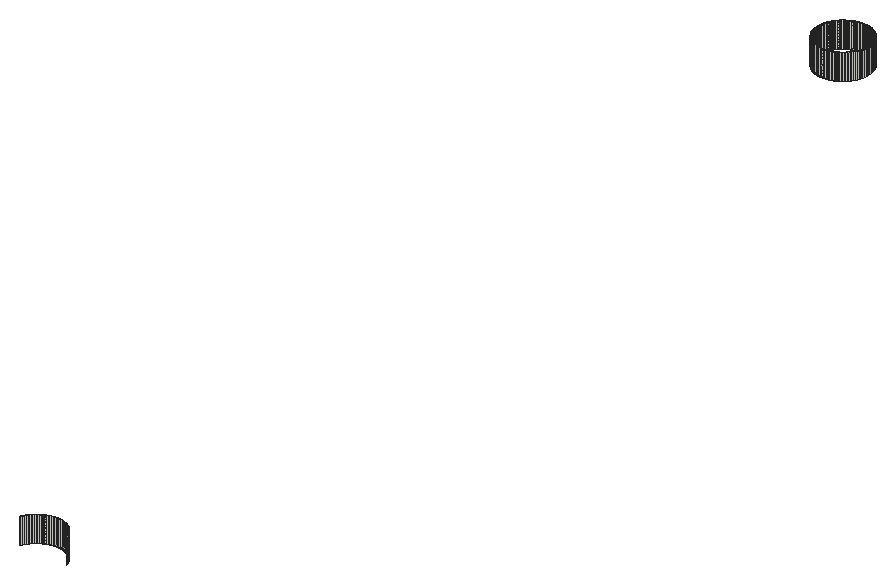
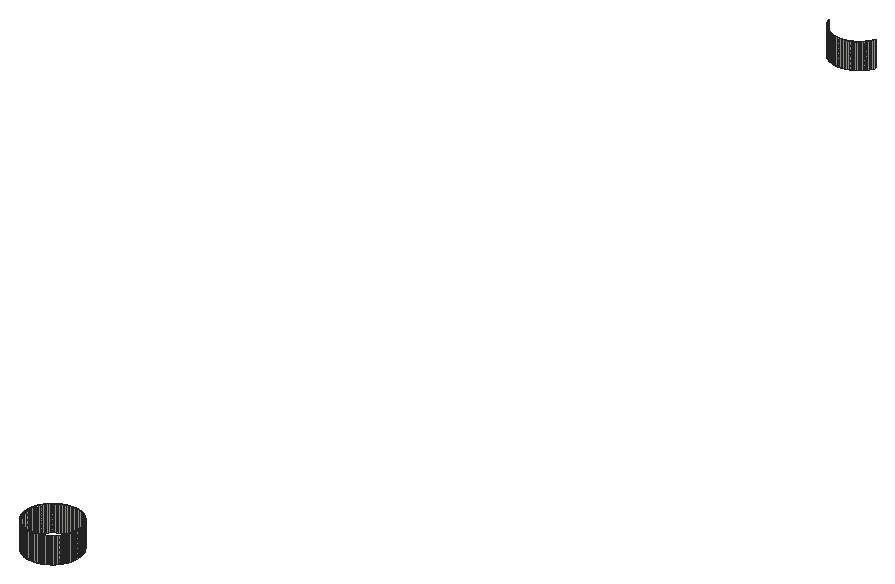
# SketchUp Ruby script. Lengths in inches.
U = 1.inch
M = Sketchup.active_model
def pt(a) = Geom::Point3d.new(a.map { |v| v * U })
def face(e, loops, mat)
  f = e.add_face(loops[0].map { |a| pt(a) })
  loops[1..].each { |l| e.add_face(l.map { |a| pt(a) }).erase! }
  f.material = f.back_material = mat if mat
  f
end
# faces: each face lists its corners as indices into pts; further lists are holes
def faces(e, pts, list, mat = nil) = list.each { |f| face(e, (f[0].is_a?(Array) ? f : [f]).map { |l| l.map { |i| pts[i] } }, mat) }
# xy, xz, yz: faces in a plane at the given z, y or x. An outline is a flat list of corners, or four numbers for a rectangle; further outlines are holes
def ring(l) = l.size == 4 ? [[l[0], l[1]], [l[2], l[1]], [l[2], l[3]], [l[0], l[3]]] : l.each_slice(2).to_a
def flat(e, list, mat, &to3) = list.each { |f| face(e, (f[0].is_a?(Array) ? f : [f]).map { |l| ring(l).map { |u, v| to3.(u, v) } }, mat) }
def xy(e, z, list, mat = nil) = flat(e, list, mat) { |x, y| [x, y, z] }
def xz(e, y, list, mat = nil) = flat(e, list, mat) { |x, z| [x, y, z] }
def yz(e, x, list, mat = nil) = flat(e, list, mat) { |y, z| [x, y, z] }
def lines(e, pts, list) = list.each { |a, b| e.add_line(pt(pts[a]), pt(pts[b])) }
# prism: a flat outline (further loops are holes) pulled along v
def prism(e, loops, v, mat = nil)
  f = face(e, loops, mat); d = Geom::Vector3d.new(v.map { |x| x * U })
  f.pushpull(f.normal.samedirection?(d) ? d.length : -d.length)
end
def box(e, o, s, mat = nil) = prism(e, [[o, [o[0] + s[0], o[1], o[2]], [o[0] + s[0], o[1] + s[1], o[2]], [o[0], o[1] + s[1], o[2]]]], [0, 0, s[2]], mat)
def at(x, y, z, deg = 0) = Geom::Transformation.translation(pt([x, y, z])) * Geom::Transformation.rotation(ORIGIN, Z_AXIS, deg.degrees)
def axes(o, x, y, z) = Geom::Transformation.new([*x, 0, *y, 0, *z, 0, *pt(o).to_a, 1])
def part(name) = M.definitions.add(name)
# library, detail: a bought-in or finely detailed component or shape, given as its bounding box
def library(name, o, s) = part(name).tap { |d| box(d.entities, o, s) }
def detail(e, o, s) = box(e.add_group.entities, o, s)
def put(e, d, t, mat = nil) = e.add_instance(d, t).tap { |i| i.material = mat if mat }
def group(e, t, mat = nil) = e.add_group.tap { |g| g.transformation = t; g.material = mat if mat }.entities
root = M.entities
xz(root,416.82,[[28.6875,258,28.76,261],[29.24,258,29.3125,261]])
xz(root,416.83,[[28.84,258,28.92,261],[28.92,258,29,261],[29,258,29.08,261],[29.08,258,29.16,261]])
xz(root,529,[[28.84,258,28.92,261],[28.92,258,29,261],[29,258,29.08,261],[29.08,258,29.16,261]])
xz(root,535,[[28.84,258,28.92,261],[28.92,258,29,261],[29,258,29.08,261],[29.08,258,29.16,261]])
yz(root,26,[[531.84,258,531.92,261],[531.92,258,532,261],[532,258,532.08,261],[532.08,258,532.16,261]])
yz(root,32,[[531.84,258,531.92,261],[531.92,258,532,261],[532,258,532.08,261],[532.08,258,532.16,261]])
p = [[31.8,414.91,258],[31.83,414.83,258],[31.83,414.83,261],[31.8,414.91,261],[26.2,414.91,258],[26.23,414.98,258],
  [26.23,414.98,261],[26.2,414.91,261],[31.77,414.98,258],[31.77,414.98,261],[26.26,415.05,258],[26.26,415.05,261],
  [31.74,415.05,258],[31.74,415.05,261],[26.29,415.125,258],[26.29,415.125,261],[26.33,415.2,258],[26.33,415.2,261],
  [31.71,415.125,258],[31.71,415.125,261],[31.67,415.2,258],[31.67,415.2,261],[26.36,415.26,258],[26.36,415.26,261],
  [31.64,415.26,258],[31.64,415.26,261],[26.4,415.33,258],[26.4,415.33,261],[26.44,415.4,258],[26.44,415.4,261],
  [31.6,415.33,258],[31.6,415.33,261],[31.56,415.4,258],[31.56,415.4,261],[26.48,415.47,258],[26.48,415.47,261],
  [31.52,415.47,258],[31.52,415.47,261],[26.53,415.53,258],[26.53,415.53,261],[26.57,415.6,258],[26.57,415.6,261],
  [31.43,415.6,258],[31.47,415.53,258],[31.47,415.53,261],[31.43,415.6,261],[26.62,415.66,258],[26.62,415.66,261],
  [31.38,415.66,258],[31.38,415.66,261],[26.67,415.72,258],[26.67,415.72,261],[26.72,415.78,258],[26.72,415.78,261],
  [31.33,415.72,258],[31.33,415.72,261],[31.28,415.78,258],[31.28,415.78,261],[26.77,415.84,258],[26.77,415.84,261],
  [26.82,415.9,258],[26.82,415.9,261],[31.23,415.84,258],[31.23,415.84,261],[31.18,415.9,258],[31.18,415.9,261],
  [26.88,415.95,258],[26.88,415.95,261],[31.12,415.95,258],[31.12,415.95,261],[26.93,416.01,258],[26.93,416.01,261],
  [26.99,416.0625,258],[26.99,416.0625,261],[31.01,416.0625,258],[31.07,416.01,258],[31.07,416.01,261],[31.01,416.0625,261],
  [27.05,416.11,258],[27.05,416.11,261],[27.11,416.16,258],[27.11,416.16,261],[30.95,416.11,258],[30.95,416.11,261],
  [30.89,416.16,258],[30.89,416.16,261],[27.17,416.21,258],[27.17,416.21,261],[27.24,416.26,258],[27.24,416.26,261],
  [30.83,416.21,258],[30.83,416.21,261],[30.76,416.26,258],[30.76,416.26,261],[27.3,416.31,258],[27.3,416.31,261],
  [27.37,416.35,258],[27.37,416.35,261],[27.43,416.39,258],[27.43,416.39,261],[30.63,416.35,258],[30.7,416.31,258],
  [30.7,416.31,261],[30.63,416.35,261],[30.57,416.39,258],[30.57,416.39,261],[27.5,416.43,258],[27.5,416.43,261],
  [27.57,416.47,258],[27.57,416.47,261],[30.43,416.47,258],[30.5,416.43,258],[30.5,416.43,261],[30.43,416.47,261],
  [27.64,416.51,258],[27.64,416.51,261],[27.71,416.54,258],[27.71,416.54,261],[27.78,416.57,258],[27.78,416.57,261],
  [30.22,416.57,258],[30.29,416.54,258],[30.29,416.54,261],[30.22,416.57,261],[30.36,416.51,258],[30.36,416.51,261],
  [27.85,416.6,258],[27.85,416.6,261],[27.92,416.63,258],[27.92,416.63,261],[28,416.66,258],[28,416.66,261],
  [30,416.66,258],[30.08,416.63,258],[30.08,416.63,261],[30,416.66,261],[30.15,416.6,258],[30.15,416.6,261],
  [28.07,416.6875,258],[28.07,416.6875,261],[28.15,416.71,258],[28.15,416.71,261],[28.22,416.73,258],[28.22,416.73,261],
  [28.3,416.75,258],[28.3,416.75,261],[29.7,416.75,258],[29.78,416.73,258],[29.78,416.73,261],[29.7,416.75,261],
  [29.85,416.71,258],[29.85,416.71,261],[29.93,416.6875,258],[29.93,416.6875,261],[28.375,416.77,258],[28.375,416.77,261],
  [28.45,416.78,258],[28.45,416.78,261],[28.53,416.8,258],[28.53,416.8,261],[28.61,416.81,258],[28.61,416.81,261],
  [28.6875,416.82,258],[28.6875,416.82,261],[28.76,416.82,258],[28.84,416.83,258],[28.84,416.83,261],[28.76,416.82,261],
  [29.16,416.83,258],[29.24,416.82,258],[29.24,416.82,261],[29.16,416.83,261],[29.3125,416.82,258],[29.39,416.81,258],
  [29.39,416.81,261],[29.3125,416.82,261],[29.47,416.8,258],[29.47,416.8,261],[29.55,416.78,258],[29.625,416.77,258],
  [29.625,416.77,261],[29.55,416.78,261],[28.61,529.03,258],[28.53,529.04,258],[28.53,529.04,261],[28.61,529.03,261],
  [28.45,529.05,258],[28.45,529.05,261],[28.6875,529.02,258],[28.6875,529.02,261],[28.76,529.01,258],[28.76,529.01,261],
  [28.84,529,258],[28.84,529,261],[29.24,529.01,258],[29.16,529,258],[29.16,529,261],[29.24,529.01,261],
  [29.3125,529.02,258],[29.3125,529.02,261],[29.39,529.03,258],[29.39,529.03,261],[29.47,529.04,258],[29.47,529.04,261],
  [29.55,529.05,258],[29.55,529.05,261],[28.07,529.15,258],[28,529.17,258],[28,529.17,261],[28.07,529.15,261],
  [28.22,529.1,258],[28.15,529.125,258],[28.15,529.125,261],[28.22,529.1,261],[28.3,529.08,258],[28.3,529.08,261],
  [28.375,529.07,258],[28.375,529.07,261],[29.625,529.07,258],[29.625,529.07,261],[29.7,529.08,258],[29.7,529.08,261],
  [29.78,529.1,258],[29.78,529.1,261],[29.85,529.125,258],[29.85,529.125,261],[29.93,529.15,258],[29.93,529.15,261],
  [30,529.17,258],[30,529.17,261],[27.85,529.23,258],[27.78,529.26,258],[27.78,529.26,261],[27.85,529.23,261],
  [27.92,529.2,258],[27.92,529.2,261],[30.08,529.2,258],[30.08,529.2,261],[30.15,529.23,258],[30.15,529.23,261],
  [30.22,529.26,258],[30.22,529.26,261],[27.71,529.29,258],[27.64,529.33,258],[27.64,529.33,261],[27.71,529.29,261],
  [27.57,529.36,258],[27.57,529.36,261],[30.29,529.29,258],[30.29,529.29,261],[30.36,529.33,258],[30.36,529.33,261],
  [30.43,529.36,258],[30.43,529.36,261],[27.5,529.4,258],[27.43,529.44,258],[27.43,529.44,261],[27.5,529.4,261],
  [27.37,529.48,258],[27.37,529.48,261],[30.5,529.4,258],[30.5,529.4,261],[30.57,529.44,258],[30.57,529.44,261],
  [30.63,529.48,258],[30.63,529.48,261],[27.3,529.53,258],[27.24,529.57,258],[27.24,529.57,261],[27.3,529.53,261],
  [30.7,529.53,258],[30.7,529.53,261],[30.76,529.57,258],[30.76,529.57,261],[27.17,529.62,258],[27.11,529.67,258],
  [27.11,529.67,261],[27.17,529.62,261],[30.83,529.62,258],[30.83,529.62,261],[30.89,529.67,258],[30.89,529.67,261],
  [27.05,529.72,258],[26.99,529.77,258],[26.99,529.77,261],[27.05,529.72,261],[30.95,529.72,258],[30.95,529.72,261],
  [31.01,529.77,258],[31.01,529.77,261],[26.93,529.82,258],[26.93,529.82,261],[26.88,529.88,258],[26.88,529.88,261],
  [31.07,529.82,258],[31.07,529.82,261],[31.12,529.88,258],[31.12,529.88,261],[26.82,529.93,258],[26.82,529.93,261],
  [26.77,529.99,258],[26.77,529.99,261],[31.18,529.93,258],[31.18,529.93,261],[31.23,529.99,258],[31.23,529.99,261],
  [26.72,530.05,258],[26.72,530.05,261],[31.28,530.05,258],[31.28,530.05,261],[26.67,530.11,258],[26.62,530.17,258],
  [26.62,530.17,261],[26.67,530.11,261],[31.33,530.11,258],[31.33,530.11,261],[31.38,530.17,258],[31.38,530.17,261],
  [26.57,530.24,258],[26.53,530.3,258],[26.53,530.3,261],[26.57,530.24,261],[31.43,530.24,258],[31.43,530.24,261],
  [31.47,530.3,258],[31.47,530.3,261],[26.48,530.37,258],[26.48,530.37,261],[31.52,530.37,258],[31.52,530.37,261],
  [26.44,530.43,258],[26.44,530.43,261],[26.4,530.5,258],[26.4,530.5,261],[31.56,530.43,258],[31.56,530.43,261],
  [31.6,530.5,258],[31.6,530.5,261],[26.36,530.57,258],[26.36,530.57,261],[31.64,530.57,258],[31.64,530.57,261],
  [26.33,530.64,258],[26.33,530.64,261],[26.29,530.71,258],[26.29,530.71,261],[31.67,530.64,258],[31.67,530.64,261],
  [31.71,530.71,258],[31.71,530.71,261],[26.26,530.78,258],[26.26,530.78,261],[31.74,530.78,258],[31.74,530.78,261],
  [26.23,530.85,258],[26.23,530.85,261],[31.77,530.85,258],[31.77,530.85,261],[26.2,530.92,258],[26.2,530.92,261],
  [26.17,531,258],[26.17,531,261],[31.8,530.92,258],[31.8,530.92,261],[31.83,531,258],[31.83,531,261],
  [26.15,531.07,258],[26.15,531.07,261],[31.85,531.07,258],[31.85,531.07,261],[26.125,531.15,258],[26.125,531.15,261],
  [26.1,531.22,258],[26.1,531.22,261],[31.875,531.15,258],[31.875,531.15,261],[31.9,531.22,258],[31.9,531.22,261],
  [26.08,531.3,258],[26.08,531.3,261],[31.92,531.3,258],[31.92,531.3,261],[26.07,531.375,258],[26.07,531.375,261],
  [31.93,531.375,258],[31.93,531.375,261],[26.05,531.45,258],[26.05,531.45,261],[31.95,531.45,258],[31.95,531.45,261],
  [26.04,531.53,258],[26.04,531.53,261],[26.03,531.61,258],[26.03,531.61,261],[31.96,531.53,258],[31.96,531.53,261],
  [31.97,531.61,258],[31.97,531.61,261],[26.02,531.6875,258],[26.02,531.6875,261],[31.98,531.6875,258],[31.98,531.6875,261],
  [26.01,531.76,258],[26.01,531.76,261],[31.99,531.76,258],[31.99,531.76,261],[26,531.84,258],[26,531.84,261],
  [32,531.84,258],[32,531.84,261],[26,532.16,258],[26.01,532.24,258],[26.01,532.24,261],[26,532.16,261],
  [26.02,532.3125,258],[26.02,532.3125,261],[31.99,532.24,258],[32,532.16,258],[32,532.16,261],[31.99,532.24,261],
  [31.98,532.3125,258],[31.98,532.3125,261],[26.03,532.39,258],[26.03,532.39,261],[31.97,532.39,258],[31.97,532.39,261],
  [26.04,532.47,258],[26.04,532.47,261],[31.96,532.47,258],[31.96,532.47,261],[26.05,532.55,258],[26.05,532.55,261],
  [26.07,532.625,258],[26.07,532.625,261],[31.95,532.55,258],[31.95,532.55,261],[31.93,532.625,258],[31.93,532.625,261],
  [26.08,532.7,258],[26.08,532.7,261],[31.92,532.7,258],[31.92,532.7,261],[26.1,532.78,258],[26.1,532.78,261],
  [31.9,532.78,258],[31.9,532.78,261],[26.125,532.85,258],[26.125,532.85,261],[31.875,532.85,258],[31.875,532.85,261],
  [26.15,532.93,258],[26.15,532.93,261],[26.17,533,258],[26.17,533,261],[31.83,533,258],[31.85,532.93,258],
  [31.85,532.93,261],[31.83,533,261],[26.2,533.08,258],[26.2,533.08,261],[31.8,533.08,258],[31.8,533.08,261],
  [26.23,533.15,258],[26.23,533.15,261],[26.26,533.22,258],[26.26,533.22,261],[31.74,533.22,258],[31.77,533.15,258],
  [31.77,533.15,261],[31.74,533.22,261],[26.29,533.29,258],[26.29,533.29,261],[31.71,533.29,258],[31.71,533.29,261],
  [26.33,533.36,258],[26.33,533.36,261],[31.67,533.36,258],[31.67,533.36,261],[26.36,533.43,258],[26.36,533.43,261],
  [26.4,533.5,258],[26.4,533.5,261],[31.64,533.43,258],[31.64,533.43,261],[31.6,533.5,258],[31.6,533.5,261],
  [26.44,533.57,258],[26.44,533.57,261],[31.56,533.57,258],[31.56,533.57,261],[26.48,533.63,258],[26.48,533.63,261],
  [26.53,533.7,258],[26.53,533.7,261],[31.52,533.63,258],[31.52,533.63,261],[31.47,533.7,258],[31.47,533.7,261],
  [26.57,533.76,258],[26.57,533.76,261],[31.43,533.76,258],[31.43,533.76,261],[26.62,533.83,258],[26.62,533.83,261],
  [26.67,533.89,258],[26.67,533.89,261],[31.33,533.89,258],[31.38,533.83,258],[31.38,533.83,261],[31.33,533.89,261],
  [26.72,533.95,258],[26.72,533.95,261],[26.77,534.01,258],[26.77,534.01,261],[31.23,534.01,258],[31.28,533.95,258],
  [31.28,533.95,261],[31.23,534.01,261],[26.82,534.07,258],[26.82,534.07,261],[31.18,534.07,258],[31.18,534.07,261],
  [26.88,534.12,258],[26.88,534.12,261],[26.93,534.18,258],[26.93,534.18,261],[31.12,534.12,258],[31.12,534.12,261],
  [31.07,534.18,258],[31.07,534.18,261],[26.99,534.23,258],[26.99,534.23,261],[27.05,534.28,258],[27.05,534.28,261],
  [30.95,534.28,258],[31.01,534.23,258],[31.01,534.23,261],[30.95,534.28,261],[27.11,534.33,258],[27.11,534.33,261],
  [27.17,534.38,258],[27.17,534.38,261],[30.83,534.38,258],[30.89,534.33,258],[30.89,534.33,261],[30.83,534.38,261],
  [27.24,534.43,258],[27.24,534.43,261],[27.3,534.47,258],[27.3,534.47,261],[30.7,534.47,258],[30.76,534.43,258],
  [30.76,534.43,261],[30.7,534.47,261],[27.37,534.52,258],[27.37,534.52,261],[27.43,534.56,258],[27.43,534.56,261],
  [30.63,534.52,258],[30.63,534.52,261],[30.57,534.56,258],[30.57,534.56,261],[27.5,534.6,258],[27.5,534.6,261],
  [27.57,534.64,258],[27.57,534.64,261],[27.64,534.67,258],[27.64,534.67,261],[30.43,534.64,258],[30.5,534.6,258],
  [30.5,534.6,261],[30.43,534.64,261],[30.36,534.67,258],[30.36,534.67,261],[27.71,534.71,258],[27.71,534.71,261],
  [27.78,534.74,258],[27.78,534.74,261],[27.85,534.77,258],[27.85,534.77,261],[30.15,534.77,258],[30.22,534.74,258],
  [30.22,534.74,261],[30.15,534.77,261],[30.29,534.71,258],[30.29,534.71,261],[27.92,534.8,258],[27.92,534.8,261],
  [28,534.83,258],[28,534.83,261],[28.07,534.85,258],[28.07,534.85,261],[29.93,534.85,258],[30,534.83,258],
  [30,534.83,261],[29.93,534.85,261],[30.08,534.8,258],[30.08,534.8,261],[28.15,534.875,258],[28.15,534.875,261],
  [28.22,534.9,258],[28.22,534.9,261],[28.3,534.92,258],[28.3,534.92,261],[28.375,534.93,258],[28.375,534.93,261],
  [28.45,534.95,258],[28.45,534.95,261],[28.53,534.96,258],[28.53,534.96,261],[29.55,534.95,258],[29.625,534.93,258],
  [29.625,534.93,261],[29.55,534.95,261],[29.47,534.96,258],[29.47,534.96,261],[29.7,534.92,258],[29.7,534.92,261],
  [29.78,534.9,258],[29.78,534.9,261],[29.85,534.875,258],[29.85,534.875,261],[28.61,534.97,258],[28.61,534.97,261],
  [28.6875,534.98,258],[28.6875,534.98,261],[28.76,534.99,258],[28.76,534.99,261],[28.84,535,258],[28.84,535,261],
  [29.24,534.99,258],[29.3125,534.98,258],[29.3125,534.98,261],[29.24,534.99,261],[29.16,535,258],[29.16,535,261],
  [29.39,534.97,258],[29.39,534.97,261]]
faces(root,p,[[0,1,2,3],[4,5,6,7],[8,0,3,9],[5,10,11,6],[12,8,9,13],[10,14,15,11],[14,16,17,15],[18,12,13,19],
  [20,18,19,21],[16,22,23,17],[24,20,21,25],[22,26,27,23],[26,28,29,27],[30,24,25,31],[32,30,31,33],[28,34,35,29],
  [36,32,33,37],[34,38,39,35],[38,40,41,39],[42,43,44,45],[43,36,37,44],[40,46,47,41],[48,42,45,49],[46,50,51,47],
  [50,52,53,51],[54,48,49,55],[56,54,55,57],[52,58,59,53],[58,60,61,59],[62,56,57,63],[64,62,63,65],[60,66,67,61],
  [68,64,65,69],[66,70,71,67],[70,72,73,71],[74,75,76,77],[75,68,69,76],[72,78,79,73],[78,80,81,79],[82,74,77,83],
  [84,82,83,85],[80,86,87,81],[86,88,89,87],[90,84,85,91],[92,90,91,93],[88,94,95,89],[94,96,97,95],[96,98,99,97],
  [100,101,102,103],[104,100,103,105],[101,92,93,102],[98,106,107,99],[106,108,109,107],[110,111,112,113],[111,104,105,112],[108,114,115,109],
  [114,116,117,115],[116,118,119,117],[120,121,122,123],[121,124,125,122],[124,110,113,125],[118,126,127,119],[126,128,129,127],[128,130,131,129],
  [132,133,134,135],[136,120,123,137],[133,136,137,134],[130,138,139,131],[138,140,141,139],[140,142,143,141],[142,144,145,143],[146,147,148,149],
  [147,150,151,148],[152,132,135,153],[150,152,153,151],[144,154,155,145],[154,156,157,155],[156,158,159,157],[158,160,161,159],[160,162,163,161],
  [164,165,166,167],[168,169,170,171],[172,173,174,175],[173,176,177,174],[178,179,180,181],[176,178,181,177],[179,146,149,180],[182,183,184,185],
  [183,186,187,184],[188,182,185,189],[190,188,189,191],[192,190,191,193],[194,195,196,197],[198,194,197,199],[200,198,199,201],[202,200,201,203],
  [204,202,203,205],[206,207,208,209],[210,211,212,213],[211,206,209,212],[214,210,213,215],[216,214,215,217],[186,216,217,187],[218,204,205,219],
  [220,218,219,221],[222,220,221,223],[224,222,223,225],[226,224,225,227],[228,226,227,229],[230,231,232,233],[207,234,235,208],[234,230,233,235],
  [236,228,229,237],[238,236,237,239],[240,238,239,241],[242,243,244,245],[243,246,247,244],[231,242,245,232],[248,240,241,249],[250,248,249,251],
  [252,250,251,253],[254,255,256,257],[255,258,259,256],[246,254,257,247],[260,252,253,261],[262,260,261,263],[264,262,263,265],[266,267,268,269],
  [258,266,269,259],[270,264,265,271],[272,270,271,273],[274,275,276,277],[267,274,277,268],[278,272,273,279],[280,278,279,281],[282,283,284,285],
  [275,282,285,276],[286,280,281,287],[288,286,287,289],[283,290,291,284],[290,292,293,291],[294,288,289,295],[296,294,295,297],[292,298,299,293],
  [298,300,301,299],[302,296,297,303],[304,302,303,305],[300,306,307,301],[308,304,305,309],[310,311,312,313],[306,310,313,307],[314,308,309,315],
  [316,314,315,317],[318,319,320,321],[311,318,321,312],[322,316,317,323],[324,322,323,325],[319,326,327,320],[328,324,325,329],[326,330,331,327],
  [330,332,333,331],[334,328,329,335],[336,334,335,337],[332,338,339,333],[340,336,337,341],[338,342,343,339],[342,344,345,343],[346,340,341,347],
  [348,346,347,349],[344,350,351,345],[352,348,349,353],[350,354,355,351],[356,352,353,357],[354,358,359,355],[358,360,361,359],[362,356,357,363],
  [364,362,363,365],[360,366,367,361],[368,364,365,369],[366,370,371,367],[370,372,373,371],[374,368,369,375],[376,374,375,377],[372,378,379,373],
  [380,376,377,381],[378,382,383,379],[384,380,381,385],[382,386,387,383],[388,384,385,389],[386,390,391,387],[390,392,393,391],[394,388,389,395],
  [396,394,395,397],[392,398,399,393],[400,396,397,401],[398,402,403,399],[404,400,401,405],[402,406,407,403],[408,404,405,409],[410,411,412,413],
  [411,414,415,412],[416,417,418,419],[420,416,419,421],[414,422,423,415],[424,420,421,425],[422,426,427,423],[428,424,425,429],[426,430,431,427],
  [430,432,433,431],[434,428,429,435],[436,434,435,437],[432,438,439,433],[440,436,437,441],[438,442,443,439],[444,440,441,445],[442,446,447,443],
  [448,444,445,449],[446,450,451,447],[450,452,453,451],[454,455,456,457],[455,448,449,456],[452,458,459,453],[460,454,457,461],[458,462,463,459],
  [462,464,465,463],[466,467,468,469],[467,460,461,468],[464,470,471,465],[472,466,469,473],[470,474,475,471],[476,472,473,477],[474,478,479,475],
  [478,480,481,479],[482,476,477,483],[484,482,483,485],[480,486,487,481],[488,484,485,489],[486,490,491,487],[490,492,493,491],[494,488,489,495],
  [496,494,495,497],[492,498,499,493],[500,496,497,501],[498,502,503,499],[502,504,505,503],[506,507,508,509],[507,500,501,508],[504,510,511,505],
  [510,512,513,511],[514,515,516,517],[515,506,509,516],[512,518,519,513],[520,514,517,521],[518,522,523,519],[522,524,525,523],[526,520,521,527],
  [528,526,527,529],[524,530,531,525],[530,532,533,531],[534,535,536,537],[535,528,529,536],[532,538,539,533],[538,540,541,539],[542,543,544,545],
  [543,534,537,544],[540,546,547,541],[546,548,549,547],[550,551,552,553],[551,542,545,552],[548,554,555,549],[554,556,557,555],[558,550,553,559],
  [560,558,559,561],[556,562,563,557],[562,564,565,563],[564,566,567,565],[568,569,570,571],[572,568,571,573],[569,560,561,570],[566,574,575,567],
  [574,576,577,575],[576,578,579,577],[580,581,582,583],[581,584,585,582],[584,572,573,585],[578,586,587,579],[586,588,589,587],[588,590,591,589],
  [592,593,594,595],[593,596,597,594],[596,580,583,597],[590,598,599,591],[598,600,601,599],[600,602,603,601],[602,604,605,603],[604,606,607,605],
  [606,608,609,607],[610,611,612,613],[614,610,613,615],[611,616,617,612],[616,618,619,617],[618,620,621,619],[620,592,595,621],[608,622,623,609],
  [622,624,625,623],[624,626,627,625],[626,628,629,627],[630,631,632,633],[634,630,633,635],[631,636,637,632],[636,614,615,637]])
